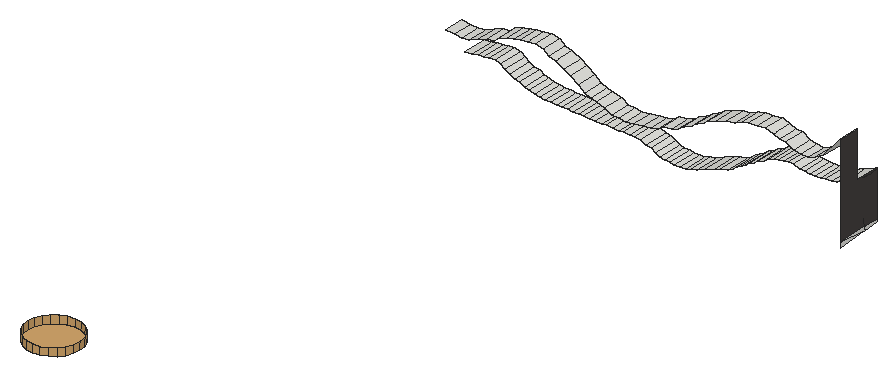
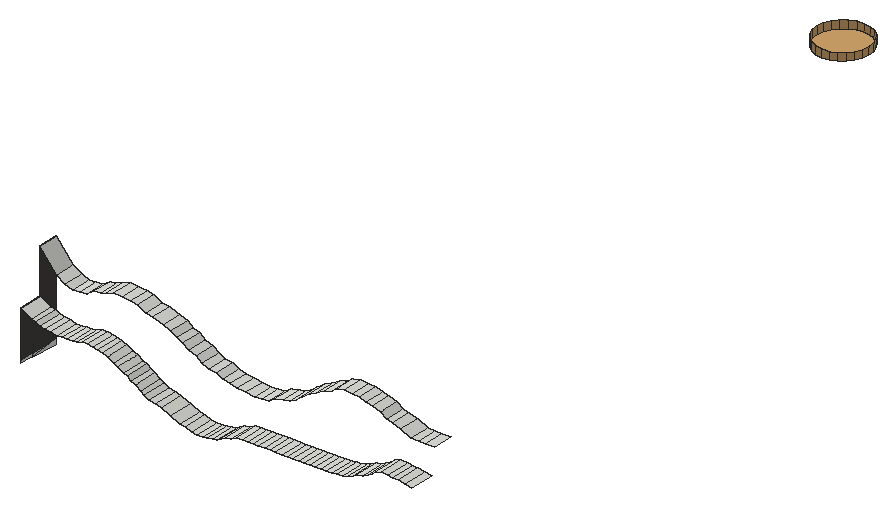
# SketchUp Ruby script. Lengths in inches.
U = 1.inch
M = Sketchup.active_model
def pt(a) = Geom::Point3d.new(a.map { |v| v * U })
def face(e, loops, mat)
  f = e.add_face(loops[0].map { |a| pt(a) })
  loops[1..].each { |l| e.add_face(l.map { |a| pt(a) }).erase! }
  f.material = f.back_material = mat if mat
  f
end
# faces: each face lists its corners as indices into pts; further lists are holes
def faces(e, pts, list, mat = nil) = list.each { |f| face(e, (f[0].is_a?(Array) ? f : [f]).map { |l| l.map { |i| pts[i] } }, mat) }
# xy, xz, yz: faces in a plane at the given z, y or x. An outline is a flat list of corners, or four numbers for a rectangle; further outlines are holes
def ring(l) = l.size == 4 ? [[l[0], l[1]], [l[2], l[1]], [l[2], l[3]], [l[0], l[3]]] : l.each_slice(2).to_a
def flat(e, list, mat, &to3) = list.each { |f| face(e, (f[0].is_a?(Array) ? f : [f]).map { |l| ring(l).map { |u, v| to3.(u, v) } }, mat) }
def xy(e, z, list, mat = nil) = flat(e, list, mat) { |x, y| [x, y, z] }
def xz(e, y, list, mat = nil) = flat(e, list, mat) { |x, z| [x, y, z] }
def yz(e, x, list, mat = nil) = flat(e, list, mat) { |y, z| [x, y, z] }
def lines(e, pts, list) = list.each { |a, b| e.add_line(pt(pts[a]), pt(pts[b])) }
# prism: a flat outline (further loops are holes) pulled along v
def prism(e, loops, v, mat = nil)
  f = face(e, loops, mat); d = Geom::Vector3d.new(v.map { |x| x * U })
  f.pushpull(f.normal.samedirection?(d) ? d.length : -d.length)
end
def box(e, o, s, mat = nil) = prism(e, [[o, [o[0] + s[0], o[1], o[2]], [o[0] + s[0], o[1] + s[1], o[2]], [o[0], o[1] + s[1], o[2]]]], [0, 0, s[2]], mat)
def at(x, y, z, deg = 0) = Geom::Transformation.translation(pt([x, y, z])) * Geom::Transformation.rotation(ORIGIN, Z_AXIS, deg.degrees)
def axes(o, x, y, z) = Geom::Transformation.new([*x, 0, *y, 0, *z, 0, *pt(o).to_a, 1])
def part(name) = M.definitions.add(name)
# library, detail: a bought-in or finely detailed component or shape, given as its bounding box
def library(name, o, s) = part(name).tap { |d| box(d.entities, o, s) }
def detail(e, o, s) = box(e.add_group.entities, o, s)
def put(e, d, t, mat = nil) = e.add_instance(d, t).tap { |i| i.material = mat if mat }
def group(e, t, mat = nil) = e.add_group.tap { |g| g.transformation = t; g.material = mat if mat }.entities
root = M.entities
M.materials.add("[Field Square Tile]").color = [211, 167, 108]
M.materials.add("[Granite Tile]1").color = [68, 65, 63]
xy(root,250.6875,[[377.043,492.582,376.331,492.675,375.668,492.95,375.098,493.387,374.661,493.957,374.386,494.62,374.293,495.332,374.386,496.043,374.661,496.707,375.098,497.276,375.668,497.713,376.331,497.988,377.043,498.082,377.754,497.988,378.418,497.713,378.987,497.276,379.424,496.707,379.699,496.043,379.793,495.332,379.699,494.62,379.424,493.957,378.987,493.387,378.418,492.95,377.754,492.675]],"[Field Square Tile]")
yz(root,406.845,[[561.053,240.932,561.053,241.519,564.151,241.17],[564.185,241.167,564.151,241.17,564.184,241.173],[564.151,241.17,561.053,241.519,564.144,241.519,564.184,241.173],[564.184,241.173,564.144,241.519,565.74,241.519,565.74,241.293]])
yz(root,406.845,[[561.053,241.519,561.053,251.165,563.178,251.165,563.178,246.426,565.74,246.426,565.74,241.519]],"[Granite Tile]1")
p = [[387.267,563.178,241.17],[387.267,565.74,241.17],[387.737,565.74,241.121],[387.737,563.178,241.121],[388.343,565.74,241.09],[388.343,563.178,241.09],
  [388.91,565.74,241.138],[388.91,563.178,241.138],[389.55,565.74,241.346],[389.55,563.178,241.346],[386.269,563.178,241.332],[386.269,565.74,241.332],
  [386.737,565.74,241.243],[386.737,563.178,241.243],[385.85,563.178,241.566],[385.85,565.74,241.566],[390.141,565.74,241.456],[390.141,563.178,241.456],
  [391.076,565.74,241.847],[391.076,563.178,241.847],[385.344,563.178,241.837],[385.344,565.74,241.837],[384.771,563.178,241.967],[384.771,565.74,241.967],
  [392.081,565.74,242.229],[392.081,563.178,242.229],[384.19,563.178,242.199],[384.19,565.74,242.199],[383.564,563.178,242.277],[383.564,565.74,242.277],
  [392.642,565.74,242.424],[392.642,563.178,242.424],[377.717,563.178,242.35],[377.717,565.74,242.35],[378.299,565.74,242.342],[378.299,563.178,242.342],
  [378.881,565.74,242.334],[378.881,563.178,242.334],[379.463,565.74,242.326],[379.463,563.178,242.326],[380.183,565.74,242.317],[380.183,563.178,242.317],
  [380.653,565.74,242.312],[380.653,563.178,242.312],[381.294,565.74,242.304],[381.294,563.178,242.304],[381.958,565.74,242.296],[381.958,563.178,242.296],
  [382.41,565.74,242.291],[382.41,563.178,242.291],[383.048,565.74,242.283],[383.048,563.178,242.283],[374.235,563.178,242.466],[374.235,565.74,242.466],
  [374.811,565.74,242.428],[374.811,563.178,242.428],[375.39,565.74,242.403],[375.39,563.178,242.403],[375.97,565.74,242.385],[375.97,563.178,242.385],
  [376.552,565.74,242.371],[376.552,563.178,242.371],[377.134,565.74,242.36],[377.134,563.178,242.36],[393.36,565.74,242.605],[393.36,563.178,242.605],
  [373.107,563.178,242.599],[373.107,565.74,242.599],[373.667,565.74,242.518],[373.667,563.178,242.518],[372.554,563.178,242.75],[372.554,565.74,242.75],
  [393.873,565.74,242.907],[393.873,563.178,242.907],[372.066,563.178,242.921],[372.066,565.74,242.921],[371.575,563.178,243.216],[371.575,565.74,243.216],
  [394.245,565.74,243.144],[394.245,563.178,243.144],[394.794,565.74,243.516],[394.794,563.178,243.516],[371.027,563.178,243.332],[371.027,565.74,243.332],
  [370.482,563.178,243.589],[370.482,565.74,243.589],[395.268,565.74,243.711],[395.268,563.178,243.711],[370.001,563.178,243.88],[370.001,565.74,243.88],
  [395.599,565.74,244.02],[395.599,563.178,244.02],[369.624,563.178,244.194],[369.624,565.74,244.194],[365.836,563.178,243.992],[365.836,565.74,243.992],
  [366.539,565.74,244.076],[366.539,563.178,244.076],[396.043,565.74,244.206],[396.043,563.178,244.206],[367.238,565.74,244.207],[367.238,563.178,244.207],
  [367.823,565.74,244.266],[367.823,563.178,244.266],[369.027,563.178,244.387],[369.027,565.74,244.387],[396.632,565.74,244.569],[396.632,563.178,244.569],
  [368.364,565.74,244.296],[368.364,563.178,244.296],[397.102,565.74,244.757],[397.102,563.178,244.757],[397.719,565.74,245.125],[397.719,563.178,245.125],
  [382.915,561.053,245.064],[382.915,563.178,245.064],[383.625,563.178,244.949],[383.625,561.053,244.949],[384.339,563.178,244.867],[384.339,561.053,244.867],
  [385.245,563.178,245.007],[385.245,561.053,245.007],[386.189,563.178,245.121],[386.189,561.053,245.121],[382.202,561.053,245.459],[382.202,563.178,245.459],
  [386.954,563.178,245.254],[386.954,561.053,245.254],[398.223,565.74,245.32],[398.223,563.178,245.32],[401.924,563.178,245.272],[401.924,565.74,245.272],
  [402.482,565.74,245.235],[402.482,563.178,245.235],[403.036,565.74,245.216],[403.036,563.178,245.216],[403.601,565.74,245.34],[403.601,563.178,245.34],
  [387.706,563.178,245.41],[387.706,561.053,245.41],[398.705,565.74,245.411],[398.705,563.178,245.411],[400.271,563.178,245.552],[400.271,565.74,245.552],
  [400.879,565.74,245.346],[400.879,563.178,245.346],[401.373,565.74,245.309],[401.373,563.178,245.309],[404.233,565.74,245.423],[404.233,563.178,245.423],
  [388.34,563.178,245.775],[388.34,561.053,245.775],[399.253,565.74,245.481],[399.253,563.178,245.481],[404.811,565.74,245.516],[404.811,563.178,245.516],
  [381.327,561.053,245.671],[381.327,563.178,245.671],[399.735,565.74,245.59],[399.735,563.178,245.59],[405.191,565.74,245.763],[405.191,563.178,245.763],
  [380.652,561.053,245.834],[380.652,563.178,245.834],[380.064,561.053,246.129],[380.064,563.178,246.129],[389.136,563.178,245.88],[389.136,561.053,245.88],
  [405.66,565.74,245.896],[405.66,563.178,245.896],[389.849,563.178,246.16],[389.849,561.053,246.16],[406.845,565.74,246.426],[406.845,563.178,246.426],
  [379.433,561.053,246.633],[379.433,563.178,246.633],[390.446,563.178,246.573],[390.446,561.053,246.573],[378.619,561.053,247.185],[378.619,563.178,247.185],
  [391.236,563.178,246.902],[391.236,561.053,246.902],[366.442,561.053,246.79],[366.442,563.178,246.79],[367.221,563.178,246.747],[367.221,561.053,246.747],
  [367.968,563.178,246.831],[367.968,561.053,246.831],[365.488,561.053,246.838],[365.488,563.178,246.838],[369.01,563.178,247.251],[369.01,561.053,247.251],
  [391.838,563.178,247.347],[391.838,561.053,247.347],[377.907,561.053,247.553],[377.907,563.178,247.553],[369.884,563.178,247.546],[369.884,561.053,247.546],
  [392.512,563.178,247.615],[392.512,561.053,247.615],[370.546,563.178,247.657],[370.546,561.053,247.657],[377.016,561.053,248.059],[377.016,563.178,248.059],
  [393.099,563.178,248.057],[393.099,561.053,248.057],[371.179,563.178,248.162],[371.179,561.053,248.162],[376.325,561.053,248.257],[376.325,563.178,248.257],
  [393.864,563.178,248.322],[393.864,561.053,248.322],[371.973,563.178,248.408],[371.973,561.053,248.408],[402.661,561.053,248.295],[402.661,563.178,248.295],
  [403.37,563.178,248.218],[403.37,561.053,248.218],[404.187,563.178,248.558],[404.187,561.053,248.558],[375.794,561.053,248.687],[375.794,563.178,248.687],
  [394.975,563.178,248.655],[394.975,561.053,248.655],[401.95,561.053,248.42],[401.95,563.178,248.42],[372.672,563.178,248.521],[372.672,561.053,248.521],
  [401.153,561.053,248.895],[401.153,563.178,248.895],[373.366,563.178,248.723],[373.366,561.053,248.723],[405.122,563.178,249.022],[405.122,561.053,249.022],
  [374.065,563.178,248.801],[374.065,561.053,248.801],[374.962,561.053,248.851],[374.962,563.178,248.851],[395.748,563.178,248.795],[395.748,561.053,248.795],
  [396.611,563.178,249.194],[396.611,561.053,249.194],[400.449,561.053,248.962],[400.449,563.178,248.962],[399.81,561.053,249.206],[399.81,563.178,249.206],
  [406.845,563.178,251.165],[406.845,561.053,251.165],[397.284,563.178,249.323],[397.284,561.053,249.323],[399.065,561.053,249.478],[399.065,563.178,249.478],
  [398.207,563.178,249.406],[398.207,561.053,249.406],[377.043,492.582,251.5],[376.331,492.675,251.5],[376.331,492.675,250.6875],[377.043,492.582,250.6875],
  [377.754,492.675,251.5],[377.754,492.675,250.6875],[375.668,492.95,251.5],[375.668,492.95,250.6875],[378.418,492.95,251.5],[378.418,492.95,250.6875],
  [375.098,493.387,251.5],[375.098,493.387,250.6875],[378.987,493.387,251.5],[378.987,493.387,250.6875],[374.661,493.957,251.5],[374.661,493.957,250.6875],
  [379.424,493.957,251.5],[379.424,493.957,250.6875],[374.386,494.62,251.5],[374.386,494.62,250.6875],[379.699,494.62,251.5],[379.699,494.62,250.6875],
  [374.293,495.332,251.5],[374.293,495.332,250.6875],[379.793,495.332,251.5],[379.793,495.332,250.6875],[374.386,496.043,251.5],[374.386,496.043,250.6875],
  [379.699,496.043,251.5],[379.699,496.043,250.6875],[374.661,496.707,251.5],[374.661,496.707,250.6875],[379.424,496.707,251.5],[379.424,496.707,250.6875],
  [375.098,497.276,251.5],[375.098,497.276,250.6875],[378.987,497.276,251.5],[378.987,497.276,250.6875],[375.668,497.713,251.5],[375.668,497.713,250.6875],
  [378.418,497.713,251.5],[378.418,497.713,250.6875],[376.331,497.988,251.5],[376.331,497.988,250.6875],[377.754,497.988,251.5],[377.754,497.988,250.6875],
  [377.043,498.082,251.5],[377.043,498.082,250.6875],[406.845,564.963,246.171],[406.845,563.948,246.265],[406.845,565.74,246.273],[406.845,564.144,241.519],
  [406.845,564.042,242.384]]
faces(root,p,[[0,1,2,3],[3,2,4,5],[5,4,6,7],[7,6,8,9],[10,11,12,13],[13,12,1,0],[14,15,11,10],[9,8,16,17],
  [17,16,18,19],[20,21,15,14],[22,23,21,20],[19,18,24,25],[26,27,23,22],[28,29,27,26],[25,24,30,31],[32,33,34,35],
  [35,34,36,37],[37,36,38,39],[39,38,40,41],[41,40,42,43],[43,42,44,45],[45,44,46,47],[47,46,48,49],[49,48,50,51],
  [51,50,29,28],[52,53,54,55],[55,54,56,57],[57,56,58,59],[59,58,60,61],[61,60,62,63],[63,62,33,32],[31,30,64,65],
  [66,67,68,69],[69,68,53,52],[70,71,67,66],[65,64,72,73],[74,75,71,70],[76,77,75,74],[73,72,78,79],[79,78,80,81],
  [82,83,77,76],[84,85,83,82],[81,80,86,87],[88,89,85,84],[87,86,90,91],[92,93,89,88],[94,95,96,97],[91,90,98,99],
  [97,96,100,101],[101,100,102,103],[104,105,93,92],[99,98,106,107],[103,102,108,109],[109,108,105,104],[107,106,110,111],[111,110,112,113],
  [114,115,116,117],[117,116,118,119],[119,118,120,121],[121,120,122,123],[124,125,115,114],[123,122,126,127],[113,112,128,129],[130,131,132,133],
  [133,132,134,135],[135,134,136,137],[127,126,138,139],[129,128,140,141],[142,143,144,145],[145,144,146,147],[147,146,131,130],[137,136,148,149],
  [139,138,150,151],[141,140,152,153],[149,148,154,155],[156,157,125,124],[153,152,158,159],[155,154,160,161],[159,158,143,142],[162,163,157,156],
  [164,165,163,162],[151,150,166,167],[161,160,168,169],[167,166,170,171],[169,168,172,173],[174,175,165,164],[171,170,176,177],[178,179,175,174],
  [177,176,180,181],[182,183,184,185],[185,184,186,187],[188,189,183,182],[187,186,190,191],[181,180,192,193],[194,195,179,178],[191,190,196,197],
  [193,192,198,199],[197,196,200,201],[202,203,195,194],[199,198,204,205],[201,200,206,207],[208,209,203,202],[205,204,210,211],[207,206,212,213],
  [214,215,216,217],[217,216,218,219],[220,221,209,208],[211,210,222,223],[224,225,215,214],[213,212,226,227],[228,229,225,224],[227,226,230,231],
  [219,218,232,233],[231,230,234,235],[236,237,221,220],[223,222,238,239],[235,234,237,236],[239,238,240,241],[242,243,229,228],[244,245,243,242],
  [233,232,246,247],[241,240,248,249],[250,251,245,244],[249,248,252,253],[253,252,251,250]])
faces(root,p,[[254,255,256,257],[258,254,257,259],[255,260,261,256],[262,258,259,263],[260,264,265,261],[266,262,263,267],[264,268,269,265],[270,266,267,271],
  [268,272,273,269],[274,270,271,275],[272,276,277,273],[278,274,275,279],[276,280,281,277],[282,278,279,283],[280,284,285,281],[286,282,283,287],
  [284,288,289,285],[290,286,287,291],[288,292,293,289],[294,290,291,295],[292,296,297,293],[298,294,295,299],[296,300,301,297],[300,298,299,301]],"[Field Square Tile]")
lines(root,p,[[302,303],[304,302],[305,306]])
